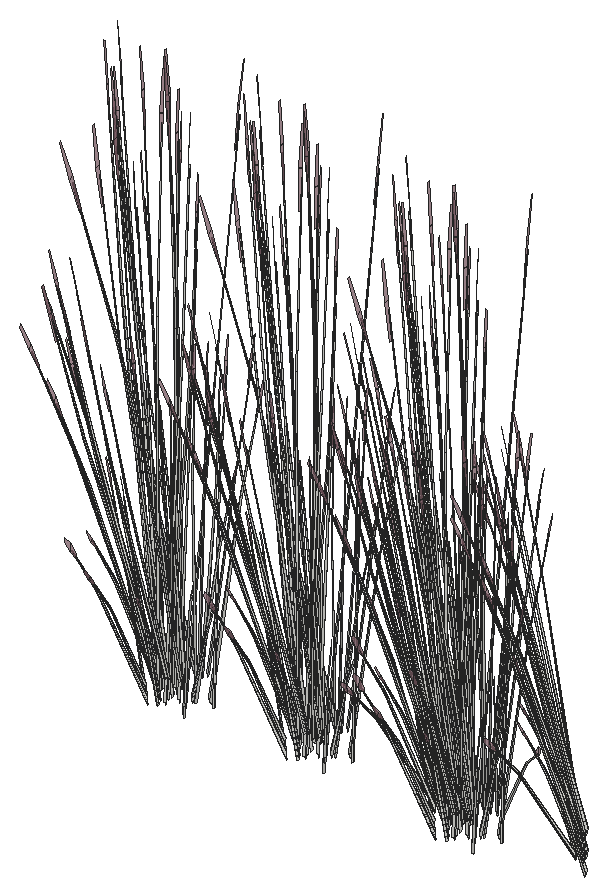
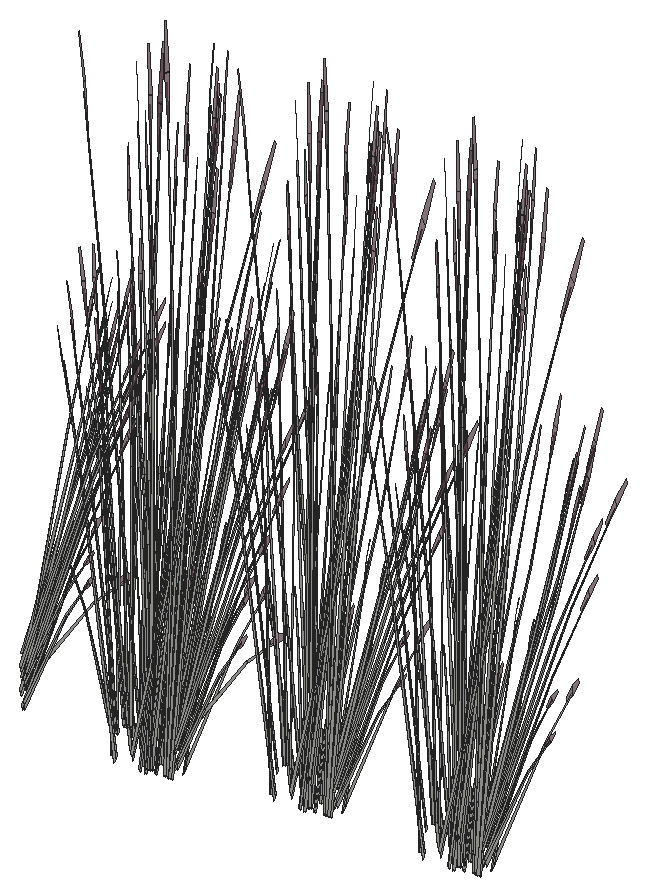
# SketchUp Ruby script. Lengths in inches.
U = 1.inch
M = Sketchup.active_model
def pt(a) = Geom::Point3d.new(a.map { |v| v * U })
def face(e, loops, mat)
  f = e.add_face(loops[0].map { |a| pt(a) })
  loops[1..].each { |l| e.add_face(l.map { |a| pt(a) }).erase! }
  f.material = f.back_material = mat if mat
  f
end
# faces: each face lists its corners as indices into pts; further lists are holes
def faces(e, pts, list, mat = nil) = list.each { |f| face(e, (f[0].is_a?(Array) ? f : [f]).map { |l| l.map { |i| pts[i] } }, mat) }
# xy, xz, yz: faces in a plane at the given z, y or x. An outline is a flat list of corners, or four numbers for a rectangle; further outlines are holes
def ring(l) = l.size == 4 ? [[l[0], l[1]], [l[2], l[1]], [l[2], l[3]], [l[0], l[3]]] : l.each_slice(2).to_a
def flat(e, list, mat, &to3) = list.each { |f| face(e, (f[0].is_a?(Array) ? f : [f]).map { |l| ring(l).map { |u, v| to3.(u, v) } }, mat) }
def xy(e, z, list, mat = nil) = flat(e, list, mat) { |x, y| [x, y, z] }
def xz(e, y, list, mat = nil) = flat(e, list, mat) { |x, z| [x, y, z] }
def yz(e, x, list, mat = nil) = flat(e, list, mat) { |y, z| [x, y, z] }
def lines(e, pts, list) = list.each { |a, b| e.add_line(pt(pts[a]), pt(pts[b])) }
# prism: a flat outline (further loops are holes) pulled along v
def prism(e, loops, v, mat = nil)
  f = face(e, loops, mat); d = Geom::Vector3d.new(v.map { |x| x * U })
  f.pushpull(f.normal.samedirection?(d) ? d.length : -d.length)
end
def box(e, o, s, mat = nil) = prism(e, [[o, [o[0] + s[0], o[1], o[2]], [o[0] + s[0], o[1] + s[1], o[2]], [o[0], o[1] + s[1], o[2]]]], [0, 0, s[2]], mat)
def at(x, y, z, deg = 0) = Geom::Transformation.translation(pt([x, y, z])) * Geom::Transformation.rotation(ORIGIN, Z_AXIS, deg.degrees)
def axes(o, x, y, z) = Geom::Transformation.new([*x, 0, *y, 0, *z, 0, *pt(o).to_a, 1])
def part(name) = M.definitions.add(name)
# library, detail: a bought-in or finely detailed component or shape, given as its bounding box
def library(name, o, s) = part(name).tap { |d| box(d.entities, o, s) }
def detail(e, o, s) = box(e.add_group.entities, o, s)
def put(e, d, t, mat = nil) = e.add_instance(d, t).tap { |i| i.material = mat if mat }
def group(e, t, mat = nil) = e.add_group.tap { |g| g.transformation = t; g.material = mat if mat }.entities
root = M.entities
M.materials.add("LightPink_Translucent").color = [144, 107, 117]
M.materials["LightPink_Translucent"].alpha = 0.75
c1 = part("blade")
p = [[2.15,0.21,22],[0,0.17,0],[0.09,0.45,0],[2.18,0.31,22],[2.29,0.31,22],[0.38,0.45,0],
  [2.48,0.24,33],[2.49,0.24,33],[2.48,0.22,33]]
faces(c1.entities,p,[[0,1,2,3],[4,5,2,3],[6,3,4,7],[8,0,3,6]])
c2 = part("seeds")
p = [[0.3,-0.1,1.38],[-0.01,-0.03,1.59],[-0.01,-0.03,0.03],[0.14,-0.07,-0.07],[0.29,-0.03,3],[0.15,0.01,3.11]]
faces(c2.entities,p,[[0,1,2,3],[1,0,4,5]],"LightPink_Translucent")
c3 = part("blade with seeds")
put(c3.entities,c1,at(0,0,0))
put(c3.entities,c2,axes([2.4,0.25,30.99],[1.5799,-0.05474,1.17369],[-0.12525,1.92788,0.29478],[-0.07173,-0.02425,1.56792]))
put(root,c3,axes([230.34,460.07,653.875],[0.20841,-0.0122,1.71376],[-0.13825,0.52864,0.13857],[-0.297,-0.0327,0.73262]))
put(root,c3,axes([230.97,459.57,654.98],[-0.50227,-0.01297,-0.71045],[0.03373,-0.54602,0.08574],[-0.21278,-0.05762,1.00501]))
put(root,c3,axes([230.56,459.71,652.59],[0.0981,0.14994,1.43002],[-0.22605,0.40756,-0.30754],[-0.23211,-0.09741,0.61141]))
put(root,c3,axes([230.74,459.22,653.875],[0.18664,0.09279,1.71376],[-0.38624,0.38925,0.13857],[-0.24072,-0.1756,0.73262]))
put(root,c3,axes([230.8,459.68,654.68],[-0.36484,0.35674,-0.51099],[-0.31952,-0.37685,-0.3958],[-0.18537,-0.05428,0.97773]))
put(root,c3,axes([230.66,459.35,654.53],[-0.28589,-0.33718,-0.35414],[0.32644,-0.31919,0.4572],[-0.16586,-0.04856,0.87481]))
put(root,c3,axes([229.98,460.16,652.77],[0.32078,-0.03854,1.1486],[-0.20348,0.33954,0.84392],[-0.15852,-0.05093,0.25299]))
put(root,c3,axes([231.84,458.93,654.98],[-0.42844,-0.2603,-0.71045],[0.30448,-0.45614,0.08574],[-0.15523,-0.15542,1.00501]))
put(root,c3,axes([231.64,458.94,654.68],[-0.4958,0.12802,-0.51099],[-0.08673,-0.48481,-0.3958],[-0.13317,-0.13893,0.97773]))
put(root,c3,axes([231,458.5,651.49],[-0.04867,0.07094,1.76342],[-0.49185,0.15296,-0.26939],[-0.11882,-0.13915,0.30037]))
put(root,c3,axes([230.69,458.77,652.13],[-0.14494,0.43975,-0.03893],[-0.4461,-0.13527,-0.17649],[-0.06773,-0.07192,0.58215]))
put(root,c3,axes([231.69,458.59,654.53],[-0.0776,-0.43378,-0.35414],[0.44361,-0.11454,0.4572],[-0.11915,-0.12431,0.87481]))
put(root,c3,axes([230.45,460.78,652.375],[-0.62828,0,0],[0,-0.6019,-0.51607],[0,-0.13709,1.63711]))
put(root,c3,axes([230.94,460.625,652.33],[-0.46736,0.45277,0.30756],[-0.46764,-0.44801,-0.36492],[-0.01632,-0.12858,1.64885]))
put(root,c3,axes([232.86,461.875,653.33],[0.4342,0.21716,1.51261],[-0.42537,0.46784,0.59816],[-0.19053,-0.27728,1.26806]))
put(root,c3,axes([231.21,457.9375,652.77],[0.2621,0.18744,1.1486],[-0.38171,0.11267,0.84392],[-0.08167,-0.14405,0.25299]))
put(root,c3,axes([232.16,461.31,652.21],[-0.30184,-0.45202,-0.44739],[0.45719,-0.31831,0.21531],[-0.09768,-0.05593,1.43643]))
put(root,c3,axes([232.21,461.57,652.4375],[0.13317,-0.63814,-0.23429],[0.63143,0.11124,0.51271],[-0.11033,-0.08813,1.5644]))
put(root,c3,axes([230.59,460.375,652.02],[0,-0.53854,-0.49651],[0.56215,0,0],[0,-0.12266,1.57504]))
put(root,c3,axes([230.83,460.875,652.48],[0,0.53854,0.49651],[-0.56215,0,0],[0,-0.12266,1.57504]))
put(root,c3,axes([232.0625,461,652.67],[-0.56585,-0.25696,-0.29095],[0.27246,-0.54236,-0.50002],[-0.01778,-0.13316,1.59708]))
put(root,c3,axes([231.81,460.45,652.1],[-0.20635,-0.55225,-0.69835],[0.59439,-0.19889,-0.18329],[-0.02281,-0.18701,1.54149]))
put(root,c3,axes([232.74,458.72,654.68],[-0.49392,-0.135,-0.51099],[0.1693,-0.46287,-0.3958],[-0.04529,-0.18636,0.97773]))
put(root,c3,axes([230.83,460.39,652.03],[0.35073,-0.33601,-0.30978],[0.35073,0.33601,0.30978],[0,-0.10823,1.38974]))
put(root,c3,axes([232.42,458.21,652.13],[-0.34721,0.30895,-0.03893],[-0.31814,-0.33837,-0.17649],[-0.0224,-0.09588,0.58215]))
put(root,c3,axes([232.96,458.43,654.53],[0.15148,-0.41415,-0.35414],[0.44193,0.12079,0.4572],[-0.04052,-0.16674,0.87481]))
put(root,c3,axes([232.22,460.67,652.36],[0.21845,0.6022,0.45755],[-0.62418,0.20941,0.17955],[0.00763,-0.11065,1.58856]))
put(root,c3,axes([232.125,460.59,652.21],[0.24378,-0.48527,-0.44739],[0.50654,0.23354,0.21531],[0,-0.11186,1.43643]))
put(root,c3,axes([232.43,460.83,652.43],[0.56613,0.26102,0.24065],[-0.27246,0.54236,0.50002],[0,-0.12502,1.60543]))
put(root,c3,axes([232.24,460.47,652.72],[-0.54562,0.03324,0.44739],[-0.04934,-0.55185,-0.21531],[0.09768,-0.05593,1.43643]))
put(root,c3,axes([231.73,458.86,652.375],[-0.31414,-0.53965,0],[0.52557,-0.30095,-0.51607],[0.1197,-0.06854,1.63711]))
put(root,c3,axes([233.04,457.56,652.77],[0.06446,0.31404,1.1486],[-0.35756,-0.17393,0.84392],[0.03848,-0.1608,0.25299]))
put(root,c3,axes([232.35,460.35,652.67],[-0.05855,-0.61451,-0.29095],[0.60981,-0.03716,-0.50002],[0.10738,-0.08185,1.59708]))
put(root,c3,axes([233.81,459.07,654.68],[-0.35968,-0.36185,-0.51099],[0.37996,-0.3169,-0.3958],[0.05473,-0.18385,0.97773]))
put(root,c3,axes([232.27,458.99,652.03],[0.46876,0.13325,-0.30978],[-0.11803,0.46926,0.30978],[0.0945,-0.05411,1.38974]))
put(root,c3,axes([232.16,458.78,652.02],[0.47024,-0.26927,-0.49651],[0.28107,0.48284,0],[0.1071,-0.06133,1.57504]))
put(root,c3,axes([234.14,458.93,654.53],[0.33997,-0.28354,-0.35414],[0.32182,0.32376,0.4572],[0.04897,-0.1645,0.87481]))
put(root,c3,axes([232.71,459.88,652.06],[0.33843,-0.40479,-0.62353],[0.42041,0.36705,-0.16365],[0.13561,-0.10098,1.37633]))
put(root,c3,axes([233.3,458.98,653.875],[-0.09355,0.18511,1.71376],[-0.39247,-0.38307,0.13857],[0.17705,-0.23875,0.73262]))
put(root,c3,axes([234.04,459,652.375],[0.31414,-0.53965,0],[0.52557,0.30095,-0.51607],[0.1197,0.06854,1.63711]))
put(root,c3,axes([234.57,458.76,651.49],[-0.0752,-0.04243,1.76342],[-0.19317,-0.47398,-0.26939],[0.13031,-0.12863,0.30037]))
put(root,c3,axes([234.55,459.9,654.68],[-0.12908,-0.49174,-0.51099],[0.48882,-0.08602,-0.3958],[0.14008,-0.13208,0.97773]))
put(root,c3,axes([235.87,460.68,652.26],[-0.31151,-0.34437,-0.06488],[0.34117,-0.31553,-0.29416],[0.09667,-0.02221,0.97024]))
put(root,c3,axes([235.15,458.92,652.77],[-0.16736,0.27414,1.1486],[-0.14385,-0.36832,0.84392],[0.13822,-0.09229,0.25299]))
put(root,c3,axes([234.91,459.95,654.53],[0.43736,-0.07697,-0.35414],[0.11549,0.43998,0.4572],[0.12533,-0.11818,0.87481]))
put(root,c3,axes([234.57,460.1,654.98],[0.26246,-0.42493,-0.71045],[0.45991,0.30199,0.08574],[0.15671,-0.15395,1.00501]))
put(root,c3,axes([234.78,460.99,654.68],[0.13612,-0.48987,-0.51099],[0.46669,0.16791,-0.3958],[0.1879,-0.04492,0.97773]))
put(root,c3,axes([234.95,459.71,652.59],[-0.1795,-0.01595,1.43002],[-0.18389,-0.42791,-0.30754],[0.22051,-0.12105,0.61141]))
put(root,c3,axes([235.28,461.13,651.98],[-0.32361,0.06463,1.41583],[-0.05151,-0.51444,0.08104],[0.22666,-0.07786,0.80566]))
put(root,c3,axes([244.23,460.07,653.875],[0.20841,-0.0122,1.71376],[-0.13825,0.52864,0.13857],[-0.297,-0.0327,0.73262]))
put(root,c3,axes([244.85,459.57,654.98],[-0.50227,-0.01297,-0.71045],[0.03373,-0.54602,0.08574],[-0.21278,-0.05762,1.00501]))
put(root,c3,axes([244.45,459.71,652.59],[0.0981,0.14994,1.43002],[-0.22605,0.40756,-0.30754],[-0.23211,-0.09741,0.61141]))
put(root,c3,axes([244.62,459.22,653.875],[0.18664,0.09279,1.71376],[-0.38624,0.38925,0.13857],[-0.24072,-0.1756,0.73262]))
put(root,c3,axes([244.69,459.68,654.68],[-0.36484,0.35674,-0.51099],[-0.31952,-0.37685,-0.3958],[-0.18537,-0.05428,0.97773]))
put(root,c3,axes([244.55,459.35,654.53],[-0.28589,-0.33718,-0.35414],[0.32644,-0.31919,0.4572],[-0.16586,-0.04856,0.87481]))
put(root,c3,axes([243.86,460.16,652.77],[0.32078,-0.03854,1.1486],[-0.20348,0.33954,0.84392],[-0.15852,-0.05093,0.25299]))
put(root,c3,axes([245.73,458.93,654.98],[-0.42844,-0.2603,-0.71045],[0.30448,-0.45614,0.08574],[-0.15523,-0.15542,1.00501]))
put(root,c3,axes([245.53,458.94,654.68],[-0.4958,0.12802,-0.51099],[-0.08673,-0.48481,-0.3958],[-0.13317,-0.13893,0.97773]))
put(root,c3,axes([244.89,458.5,651.49],[-0.04867,0.07094,1.76342],[-0.49185,0.15296,-0.26939],[-0.11882,-0.13915,0.30037]))
put(root,c3,axes([244.58,458.77,652.13],[-0.14494,0.43975,-0.03893],[-0.4461,-0.13527,-0.17649],[-0.06773,-0.07192,0.58215]))
put(root,c3,axes([245.58,458.59,654.53],[-0.0776,-0.43378,-0.35414],[0.44361,-0.11454,0.4572],[-0.11915,-0.12431,0.87481]))
put(root,c3,axes([244.34,460.78,652.375],[-0.62828,0,0],[0,-0.6019,-0.51607],[0,-0.13709,1.63711]))
put(root,c3,axes([244.83,460.625,652.33],[-0.46736,0.45277,0.30756],[-0.46764,-0.44801,-0.36492],[-0.01632,-0.12858,1.64885]))
put(root,c3,axes([246.75,461.875,653.33],[0.4342,0.21716,1.51261],[-0.42537,0.46784,0.59816],[-0.19053,-0.27728,1.26806]))
put(root,c3,axes([245.09,457.9375,652.77],[0.2621,0.18744,1.1486],[-0.38171,0.11267,0.84392],[-0.08167,-0.14405,0.25299]))
put(root,c3,axes([246.05,461.31,652.21],[-0.30184,-0.45202,-0.44739],[0.45719,-0.31831,0.21531],[-0.09768,-0.05593,1.43643]))
put(root,c3,axes([246.09,461.57,652.4375],[0.13317,-0.63814,-0.23429],[0.63143,0.11124,0.51271],[-0.11033,-0.08813,1.5644]))
put(root,c3,axes([244.48,460.375,652.02],[0,-0.53854,-0.49651],[0.56215,0,0],[0,-0.12266,1.57504]))
put(root,c3,axes([244.72,460.875,652.48],[0,0.53854,0.49651],[-0.56215,0,0],[0,-0.12266,1.57504]))
put(root,c3,axes([245.95,461,652.67],[-0.56585,-0.25696,-0.29095],[0.27246,-0.54236,-0.50002],[-0.01778,-0.13316,1.59708]))
put(root,c3,axes([245.7,460.45,652.1],[-0.20635,-0.55225,-0.69835],[0.59439,-0.19889,-0.18329],[-0.02281,-0.18701,1.54149]))
put(root,c3,axes([246.625,458.72,654.68],[-0.49392,-0.135,-0.51099],[0.1693,-0.46287,-0.3958],[-0.04529,-0.18636,0.97773]))
put(root,c3,axes([244.72,460.39,652.03],[0.35073,-0.33601,-0.30978],[0.35073,0.33601,0.30978],[0,-0.10823,1.38974]))
put(root,c3,axes([246.31,458.21,652.13],[-0.34721,0.30895,-0.03893],[-0.31814,-0.33837,-0.17649],[-0.0224,-0.09588,0.58215]))
put(root,c3,axes([246.85,458.43,654.53],[0.15148,-0.41415,-0.35414],[0.44193,0.12079,0.4572],[-0.04052,-0.16674,0.87481]))
put(root,c3,axes([246.11,460.67,652.36],[0.21845,0.6022,0.45755],[-0.62418,0.20941,0.17955],[0.00763,-0.11065,1.58856]))
put(root,c3,axes([246.01,460.59,652.21],[0.24378,-0.48527,-0.44739],[0.50654,0.23354,0.21531],[0,-0.11186,1.43643]))
put(root,c3,axes([246.3125,460.83,652.43],[0.56613,0.26102,0.24065],[-0.27246,0.54236,0.50002],[0,-0.12502,1.60543]))
put(root,c3,axes([246.13,460.47,652.72],[-0.54562,0.03324,0.44739],[-0.04934,-0.55185,-0.21531],[0.09768,-0.05593,1.43643]))
put(root,c3,axes([245.62,458.86,652.375],[-0.31414,-0.53965,0],[0.52557,-0.30095,-0.51607],[0.1197,-0.06854,1.63711]))
put(root,c3,axes([246.93,457.56,652.77],[0.06446,0.31404,1.1486],[-0.35756,-0.17393,0.84392],[0.03848,-0.1608,0.25299]))
put(root,c3,axes([246.23,460.35,652.67],[-0.05855,-0.61451,-0.29095],[0.60981,-0.03716,-0.50002],[0.10738,-0.08185,1.59708]))
put(root,c3,axes([247.69,459.07,654.68],[-0.35968,-0.36185,-0.51099],[0.37996,-0.3169,-0.3958],[0.05473,-0.18385,0.97773]))
put(root,c3,axes([246.15,458.99,652.03],[0.46876,0.13325,-0.30978],[-0.11803,0.46926,0.30978],[0.0945,-0.05411,1.38974]))
put(root,c3,axes([246.04,458.78,652.02],[0.47024,-0.26927,-0.49651],[0.28107,0.48284,0],[0.1071,-0.06133,1.57504]))
put(root,c3,axes([248.03,458.93,654.53],[0.33997,-0.28354,-0.35414],[0.32182,0.32376,0.4572],[0.04897,-0.1645,0.87481]))
put(root,c3,axes([246.6,459.88,652.06],[0.33843,-0.40479,-0.62353],[0.42041,0.36705,-0.16365],[0.13561,-0.10098,1.37633]))
put(root,c3,axes([247.18,458.98,653.875],[-0.09355,0.18511,1.71376],[-0.39247,-0.38307,0.13857],[0.17705,-0.23875,0.73262]))
put(root,c3,axes([247.93,459,652.375],[0.31414,-0.53965,0],[0.52557,0.30095,-0.51607],[0.1197,0.06854,1.63711]))
put(root,c3,axes([248.46,458.76,651.49],[-0.0752,-0.04243,1.76342],[-0.19317,-0.47398,-0.26939],[0.13031,-0.12863,0.30037]))
put(root,c3,axes([248.44,459.9,654.68],[-0.12908,-0.49174,-0.51099],[0.48882,-0.08602,-0.3958],[0.14008,-0.13208,0.97773]))
put(root,c3,axes([249.76,460.68,652.26],[-0.31151,-0.34437,-0.06488],[0.34117,-0.31553,-0.29416],[0.09667,-0.02221,0.97024]))
put(root,c3,axes([249.04,458.92,652.77],[-0.16736,0.27414,1.1486],[-0.14385,-0.36832,0.84392],[0.13822,-0.09229,0.25299]))
put(root,c3,axes([248.8,459.95,654.53],[0.43736,-0.07697,-0.35414],[0.11549,0.43998,0.4572],[0.12533,-0.11818,0.87481]))
put(root,c3,axes([248.45,460.1,654.98],[0.26246,-0.42493,-0.71045],[0.45991,0.30199,0.08574],[0.15671,-0.15395,1.00501]))
put(root,c3,axes([248.67,460.99,654.68],[0.13612,-0.48987,-0.51099],[0.46669,0.16791,-0.3958],[0.1879,-0.04492,0.97773]))
put(root,c3,axes([248.83,459.71,652.59],[-0.1795,-0.01595,1.43002],[-0.18389,-0.42791,-0.30754],[0.22051,-0.12105,0.61141]))
put(root,c3,axes([249.17,461.13,651.98],[-0.32361,0.06463,1.41583],[-0.05151,-0.51444,0.08104],[0.22666,-0.07786,0.80566]))
put(root,c3,axes([259.09,460.07,651.875],[0.20841,-0.0122,1.71376],[-0.13825,0.52864,0.13857],[-0.297,-0.0327,0.73262]))
put(root,c3,axes([259.71,459.57,652.98],[-0.50227,-0.01297,-0.71045],[0.03373,-0.54602,0.08574],[-0.21278,-0.05762,1.00501]))
put(root,c3,axes([259.31,459.71,650.59],[0.0981,0.14994,1.43002],[-0.22605,0.40756,-0.30754],[-0.23211,-0.09741,0.61141]))
put(root,c3,axes([259.48,459.22,651.875],[0.18664,0.09279,1.71376],[-0.38624,0.38925,0.13857],[-0.24072,-0.1756,0.73262]))
put(root,c3,axes([259.54,459.68,652.68],[-0.36484,0.35674,-0.51099],[-0.31952,-0.37685,-0.3958],[-0.18537,-0.05428,0.97773]))
put(root,c3,axes([259.03,458.68,652.71],[0.03725,0.05374,1.77383],[-0.17957,0.48312,-0.16761],[-0.18186,0.0035,0.31391]))
put(root,c3,axes([259.45,458.36,652.72],[-0.10811,-0.0038,1.74944],[-0.34418,0.38014,-0.27667],[-0.18364,-0.07767,0.14031]))
put(root,c3,axes([259.74,459.3125,653.03],[-0.0269,0.54769,-0.1216],[-0.50939,-0.01497,-0.67495],[-0.19618,-0.03804,1.02557]))
put(root,c3,axes([259.41,459.35,652.53],[-0.28589,-0.33718,-0.35414],[0.32644,-0.31919,0.4572],[-0.16586,-0.04856,0.87481]))
put(root,c3,axes([258.72,460.16,650.77],[0.32078,-0.03854,1.1486],[-0.20348,0.33954,0.84392],[-0.15852,-0.05093,0.25299]))
put(root,c3,axes([259.37,459.22,653.09],[0.41494,-0.39744,0.53763],[0.35786,0.42207,0.4433],[-0.19468,-0.07331,1.11249]))
put(root,c3,axes([259.56,459.22,652.73],[0.0253,-0.40952,0.0643],[0.38204,0.01123,0.50621],[-0.14634,-0.04285,0.77189]))
put(root,c3,axes([260.73,458.51,653.43],[-0.33533,0.51628,-0.13619],[-0.48563,-0.29744,-0.75594],[-0.16881,-0.14586,1.14864]))
put(root,c3,axes([259.82,459.53,653.05],[0.28589,0.33718,0.35414],[-0.32644,0.31919,-0.4572],[-0.16586,-0.04856,0.87481]))
put(root,c3,axes([260.59,458.93,652.98],[-0.42844,-0.2603,-0.71045],[0.30448,-0.45614,0.08574],[-0.15523,-0.15542,1.00501]))
put(root,c3,axes([260.38,458.94,652.68],[-0.4958,0.12802,-0.51099],[-0.08673,-0.48481,-0.3958],[-0.13317,-0.13893,0.97773]))
put(root,c3,axes([259.74,458.5,649.49],[-0.04867,0.07094,1.76342],[-0.49185,0.15296,-0.26939],[-0.11882,-0.13915,0.30037]))
put(root,c3,axes([259.4375,458.77,650.13],[-0.14494,0.43975,-0.03893],[-0.4461,-0.13527,-0.17649],[-0.06773,-0.07192,0.58215]))
put(root,c3,axes([260.6,457.28,652.71],[-0.00937,0.06455,1.77383],[-0.46231,0.23427,-0.16761],[-0.13604,-0.11975,0.31391]))
put(root,c3,axes([260.4375,458.59,652.53],[-0.0776,-0.43378,-0.35414],[0.44361,-0.11454,0.4572],[-0.11915,-0.12431,0.87481]))
put(root,c3,axes([259.2,460.78,650.375],[-0.62828,0,0],[0,-0.6019,-0.51607],[0,-0.13709,1.63711]))
put(root,c3,axes([260.7,458.94,653.05],[0.0776,0.43378,0.35414],[-0.44361,0.11454,-0.4572],[-0.11915,-0.12431,0.87481]))
put(root,c3,axes([259.6875,460.625,650.33],[-0.46736,0.45277,0.30756],[-0.46764,-0.44801,-0.36492],[-0.01632,-0.12858,1.64885]))
put(root,c3,axes([261.61,461.875,651.33],[0.4342,0.21716,1.51261],[-0.42537,0.46784,0.59816],[-0.19053,-0.27728,1.26806]))
put(root,c3,axes([259.95,457.9375,650.77],[0.2621,0.18744,1.1486],[-0.38171,0.11267,0.84392],[-0.08167,-0.14405,0.25299]))
put(root,c3,axes([260.91,461.31,650.21],[-0.30184,-0.45202,-0.44739],[0.45719,-0.31831,0.21531],[-0.09768,-0.05593,1.43643]))
put(root,c3,axes([260.5,458.43,653.09],[0.55971,-0.13842,0.53763],[0.09714,0.54299,0.4433],[-0.13164,-0.16003,1.11249]))
put(root,c3,axes([260.63,458.55,652.73],[0.22836,-0.34211,0.0643],[0.3252,0.19918,0.50621],[-0.10513,-0.10968,0.77189]))
put(root,c3,axes([260.95,461.57,650.4375],[0.13317,-0.63814,-0.23429],[0.63143,0.11124,0.51271],[-0.11033,-0.08813,1.5644]))
put(root,c3,axes([259.34,460.375,650.02],[0,-0.53854,-0.49651],[0.56215,0,0],[0,-0.12266,1.57504]))
put(root,c3,axes([259.58,460.875,650.48],[0,0.53854,0.49651],[-0.56215,0,0],[0,-0.12266,1.57504]))
put(root,c3,axes([260.81,461,650.67],[-0.56585,-0.25696,-0.29095],[0.27246,-0.54236,-0.50002],[-0.01778,-0.13316,1.59708]))
put(root,c3,axes([260.56,460.45,650.1],[-0.20635,-0.55225,-0.69835],[0.59439,-0.19889,-0.18329],[-0.02281,-0.18701,1.54149]))
put(root,c3,axes([261.91,458.7,653.03],[-0.49168,0.25073,-0.1216],[-0.24162,-0.44501,-0.67495],[-0.06487,-0.18753,1.02557]))
put(root,c3,axes([261.49,458.72,652.68],[-0.49392,-0.135,-0.51099],[0.1693,-0.46287,-0.3958],[-0.04529,-0.18636,0.97773]))
put(root,c3,axes([259.58,460.39,650.03],[0.35073,-0.33601,-0.30978],[0.35073,0.33601,0.30978],[0,-0.10823,1.38974]))
put(root,c3,axes([261.17,458.21,650.13],[-0.34721,0.30895,-0.03893],[-0.31814,-0.33837,-0.17649],[-0.0224,-0.09588,0.58215]))
put(root,c3,axes([260.86,461.14,650.72],[-0.24378,0.48527,0.44739],[-0.50654,-0.23354,-0.21531],[0,-0.11186,1.43643]))
put(root,c3,axes([261.76,458.87,653.05],[-0.15148,0.41415,0.35414],[-0.44193,-0.12079,-0.4572],[-0.04052,-0.16674,0.87481]))
put(root,c3,axes([261.71,458.43,652.53],[0.15148,-0.41415,-0.35414],[0.44193,0.12079,0.4572],[-0.04052,-0.16674,0.87481]))
put(root,c3,axes([260.97,460.67,650.36],[0.21845,0.6022,0.45755],[-0.62418,0.20941,0.17955],[0.00763,-0.11065,1.58856]))
put(root,c3,axes([260.87,460.59,650.21],[0.24378,-0.48527,-0.44739],[0.50654,0.23354,0.21531],[0,-0.11186,1.43643]))
put(root,c3,axes([261.9,458.5,652.73],[0.37023,-0.18303,0.0643],[0.18122,0.33376,0.50621],[-0.03575,-0.14712,0.77189]))
put(root,c3,axes([261.77,458.53,652.73],[0.4951,0.14079,0.48003],[-0.1693,0.46287,0.3958],[-0.02975,-0.18203,0.9933]))
put(root,c3,axes([261.17,460.83,650.43],[0.56613,0.26102,0.24065],[-0.27246,0.54236,0.50002],[0,-0.12502,1.60543]))
put(root,c3,axes([260.99,460.47,650.72],[-0.54562,0.03324,0.44739],[-0.04934,-0.55185,-0.21531],[0.09768,-0.05593,1.43643]))
put(root,c3,axes([260.48,458.86,650.375],[-0.31414,-0.53965,0],[0.52557,-0.30095,-0.51607],[0.1197,-0.06854,1.63711]))
put(root,c3,axes([261.79,457.56,650.77],[0.06446,0.31404,1.1486],[-0.35756,-0.17393,0.84392],[0.03848,-0.1608,0.25299]))
put(root,c3,axes([263.32,458.07,652.71],[-0.05103,0.04113,1.77383],[-0.49994,-0.13878,-0.16761],[-0.0181,-0.17951,0.31391]))
put(root,c3,axes([262.93,459.26,653.03],[-0.55221,-0.02668,-0.1216],[0.01509,-0.50521,-0.67495],[0.03836,-0.19458,1.02557]))
put(root,c3,axes([262.71,459.34,653.05],[-0.33997,0.28354,0.35414],[-0.32182,-0.32376,-0.4572],[0.04897,-0.1645,0.87481]))
put(root,c3,axes([261.09,460.35,650.67],[-0.05855,-0.61451,-0.29095],[0.60981,-0.03716,-0.50002],[0.10738,-0.08185,1.59708]))
put(root,c3,axes([262.55,459.07,652.68],[-0.35968,-0.36185,-0.51099],[0.37996,-0.3169,-0.3958],[0.05473,-0.18385,0.97773]))
put(root,c3,axes([261.01,458.99,650.03],[0.46876,0.13325,-0.30978],[-0.11803,0.46926,0.30978],[0.0945,-0.05411,1.38974]))
put(root,c3,axes([260.9,458.78,650.02],[0.47024,-0.26927,-0.49651],[0.28107,0.48284,0],[0.1071,-0.06133,1.57504]))
put(root,c3,axes([262.89,458.93,652.53],[0.33997,-0.28354,-0.35414],[0.32182,0.32376,0.4572],[0.04897,-0.1645,0.87481]))
put(root,c3,axes([263.02,459.08,652.73],[0.4129,0.02509,0.0643],[-0.01132,0.37891,0.50621],[0.04321,-0.14514,0.77189]))
put(root,c3,axes([261.46,459.88,650.06],[0.33843,-0.40479,-0.62353],[0.42041,0.36705,-0.16365],[0.13561,-0.10098,1.37633]))
put(root,c3,axes([262.89,459.05,652.73],[0.35779,0.36745,0.48003],[-0.37996,0.3169,0.3958],[0.066,-0.17239,0.9933]))
put(root,c3,axes([263.3,460.21,653.05],[-0.43736,0.07697,0.35414],[-0.11549,-0.43998,-0.4572],[0.12533,-0.11818,0.87481]))
put(root,c3,axes([262.04,458.98,651.875],[-0.09355,0.18511,1.71376],[-0.39247,-0.38307,0.13857],[0.17705,-0.23875,0.73262]))
put(root,c3,axes([263.53,460.25,653.03],[-0.46478,-0.29695,-0.1216],[0.26776,-0.43004,-0.67495],[0.13131,-0.14949,1.02557]))
put(root,c3,axes([262.79,459,650.375],[0.31414,-0.53965,0],[0.52557,0.30095,-0.51607],[0.1197,0.06854,1.63711]))
put(root,c3,axes([263.32,458.76,649.49],[-0.0752,-0.04243,1.76342],[-0.19317,-0.47398,-0.26939],[0.13031,-0.12863,0.30037]))
put(root,c3,axes([263.3,459.9,652.68],[-0.12908,-0.49174,-0.51099],[0.48882,-0.08602,-0.3958],[0.14008,-0.13208,0.97773]))
put(root,c3,axes([264.61,460.68,650.26],[-0.31151,-0.34437,-0.06488],[0.34117,-0.31553,-0.29416],[0.09667,-0.02221,0.97024]))
put(root,c3,axes([263.9,458.92,650.77],[-0.16736,0.27414,1.1486],[-0.14385,-0.36832,0.84392],[0.13822,-0.09229,0.25299]))
put(root,c3,axes([263.7,460.14,652.73],[0.34493,0.22649,0.0643],[-0.20082,0.32253,0.50621],[0.11059,-0.10427,0.77189]))
put(root,c3,axes([263.6,460.05,652.73],[0.12461,0.49565,0.48003],[-0.48882,0.08602,0.3958],[0.14406,-0.11657,0.9933]))
put(root,c3,axes([264.67,460.125,652.71],[-0.06563,-0.00409,1.77383],[-0.27252,-0.43825,-0.16761],[0.10944,-0.1441,0.31391]))
put(root,c3,axes([263.66,459.95,652.53],[0.43736,-0.07697,-0.35414],[0.11549,0.43998,0.4572],[0.12533,-0.11818,0.87481]))
put(root,c3,axes([263.3125,460.1,652.98],[0.26246,-0.42493,-0.71045],[0.45991,0.30199,0.08574],[0.15671,-0.15395,1.00501]))
put(root,c3,axes([263.55,461.41,653.03],[-0.25281,-0.48765,-0.1216],[0.44869,-0.23964,-0.67495],[0.18908,-0.06434,1.02557]))
put(root,c3,axes([263.53,460.99,652.68],[0.13612,-0.48987,-0.51099],[0.46669,0.16791,-0.3958],[0.1879,-0.04492,0.97773]))
put(root,c3,axes([263.69,459.71,650.59],[-0.1795,-0.01595,1.43002],[-0.18389,-0.42791,-0.30754],[0.22051,-0.12105,0.61141]))
put(root,c3,axes([264.03,461.13,649.98],[-0.32361,0.06463,1.41583],[-0.05151,-0.51444,0.08104],[0.22666,-0.07786,0.80566]))
put(root,c3,axes([264.92,460.65,652.72],[0.06972,-0.08203,1.74944],[-0.08924,-0.50318,-0.27667],[0.17494,-0.0954,0.14031]))
put(root,c3,axes([273.34,460.07,651.875],[0.20841,-0.0122,1.71376],[-0.13825,0.52864,0.13857],[-0.297,-0.0327,0.73262]))
put(root,c3,axes([273.34,460.07,653.875],[0.20841,-0.0122,1.71376],[-0.13825,0.52864,0.13857],[-0.297,-0.0327,0.73262]))
put(root,c3,axes([273.97,459.57,652.98],[-0.50227,-0.01297,-0.71045],[0.03373,-0.54602,0.08574],[-0.21278,-0.05762,1.00501]))
put(root,c3,axes([273.97,459.57,654.98],[-0.50227,-0.01297,-0.71045],[0.03373,-0.54602,0.08574],[-0.21278,-0.05762,1.00501]))
put(root,c3,axes([273.56,459.71,650.59],[0.0981,0.14994,1.43002],[-0.22605,0.40756,-0.30754],[-0.23211,-0.09741,0.61141]))
put(root,c3,axes([273.56,459.71,652.59],[0.0981,0.14994,1.43002],[-0.22605,0.40756,-0.30754],[-0.23211,-0.09741,0.61141]))
put(root,c3,axes([273.74,459.22,651.875],[0.18664,0.09279,1.71376],[-0.38624,0.38925,0.13857],[-0.24072,-0.1756,0.73262]))
put(root,c3,axes([273.74,459.22,653.875],[0.18664,0.09279,1.71376],[-0.38624,0.38925,0.13857],[-0.24072,-0.1756,0.73262]))
put(root,c3,axes([273.8,459.68,652.68],[-0.36484,0.35674,-0.51099],[-0.31952,-0.37685,-0.3958],[-0.18537,-0.05428,0.97773]))
put(root,c3,axes([273.8,459.68,654.68],[-0.36484,0.35674,-0.51099],[-0.31952,-0.37685,-0.3958],[-0.18537,-0.05428,0.97773]))
put(root,c3,axes([273.28,458.68,652.71],[0.03725,0.05374,1.77383],[-0.17957,0.48312,-0.16761],[-0.18186,0.0035,0.31391]))
put(root,c3,axes([273.7,458.36,652.72],[-0.10811,-0.0038,1.74944],[-0.34418,0.38014,-0.27667],[-0.18364,-0.07767,0.14031]))
put(root,c3,axes([273.99,459.3125,653.03],[-0.0269,0.54769,-0.1216],[-0.50939,-0.01497,-0.67495],[-0.19618,-0.03804,1.02557]))
put(root,c3,axes([273.66,459.35,652.53],[-0.28589,-0.33718,-0.35414],[0.32644,-0.31919,0.4572],[-0.16586,-0.04856,0.87481]))
put(root,c3,axes([273.66,459.35,654.53],[-0.28589,-0.33718,-0.35414],[0.32644,-0.31919,0.4572],[-0.16586,-0.04856,0.87481]))
put(root,c3,axes([272.98,460.16,650.77],[0.32078,-0.03854,1.1486],[-0.20348,0.33954,0.84392],[-0.15852,-0.05093,0.25299]))
put(root,c3,axes([272.98,460.16,652.77],[0.32078,-0.03854,1.1486],[-0.20348,0.33954,0.84392],[-0.15852,-0.05093,0.25299]))
